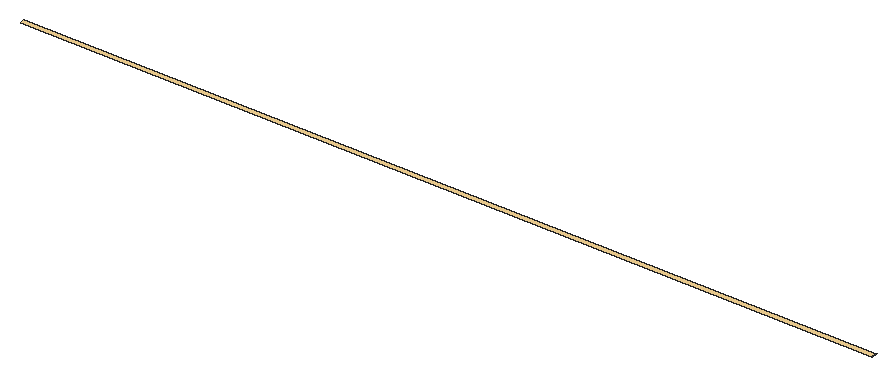
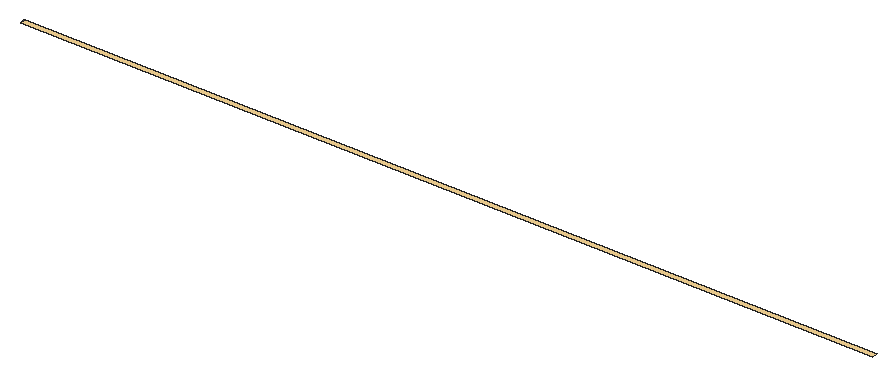
# SketchUp Ruby script. Lengths in inches.
U = 1.inch
M = Sketchup.active_model
def pt(a) = Geom::Point3d.new(a.map { |v| v * U })
def face(e, loops, mat)
  f = e.add_face(loops[0].map { |a| pt(a) })
  loops[1..].each { |l| e.add_face(l.map { |a| pt(a) }).erase! }
  f.material = f.back_material = mat if mat
  f
end
# faces: each face lists its corners as indices into pts; further lists are holes
def faces(e, pts, list, mat = nil) = list.each { |f| face(e, (f[0].is_a?(Array) ? f : [f]).map { |l| l.map { |i| pts[i] } }, mat) }
# xy, xz, yz: faces in a plane at the given z, y or x. An outline is a flat list of corners, or four numbers for a rectangle; further outlines are holes
def ring(l) = l.size == 4 ? [[l[0], l[1]], [l[2], l[1]], [l[2], l[3]], [l[0], l[3]]] : l.each_slice(2).to_a
def flat(e, list, mat, &to3) = list.each { |f| face(e, (f[0].is_a?(Array) ? f : [f]).map { |l| ring(l).map { |u, v| to3.(u, v) } }, mat) }
def xy(e, z, list, mat = nil) = flat(e, list, mat) { |x, y| [x, y, z] }
def xz(e, y, list, mat = nil) = flat(e, list, mat) { |x, z| [x, y, z] }
def yz(e, x, list, mat = nil) = flat(e, list, mat) { |y, z| [x, y, z] }
def lines(e, pts, list) = list.each { |a, b| e.add_line(pt(pts[a]), pt(pts[b])) }
# prism: a flat outline (further loops are holes) pulled along v
def prism(e, loops, v, mat = nil)
  f = face(e, loops, mat); d = Geom::Vector3d.new(v.map { |x| x * U })
  f.pushpull(f.normal.samedirection?(d) ? d.length : -d.length)
end
def box(e, o, s, mat = nil) = prism(e, [[o, [o[0] + s[0], o[1], o[2]], [o[0] + s[0], o[1] + s[1], o[2]], [o[0], o[1] + s[1], o[2]]]], [0, 0, s[2]], mat)
def at(x, y, z, deg = 0) = Geom::Transformation.translation(pt([x, y, z])) * Geom::Transformation.rotation(ORIGIN, Z_AXIS, deg.degrees)
def axes(o, x, y, z) = Geom::Transformation.new([*x, 0, *y, 0, *z, 0, *pt(o).to_a, 1])
def part(name) = M.definitions.add(name)
# library, detail: a bought-in or finely detailed component or shape, given as its bounding box
def library(name, o, s) = part(name).tap { |d| box(d.entities, o, s) }
def detail(e, o, s) = box(e.add_group.entities, o, s)
def put(e, d, t, mat = nil) = e.add_instance(d, t).tap { |i| i.material = mat if mat }
def group(e, t, mat = nil) = e.add_group.tap { |g| g.transformation = t; g.material = mat if mat }.entities
root = M.entities
M.materials.add("1432 AP 8245 TAR ROAD").color = [71, 72, 75]
M.materials.add("Outer Light").color = [251, 217, 152]
xy(root,171.29,[[537,95.37,537.16,96.87]],"1432 AP 8245 TAR ROAD")
xy(root,171.29,[[279,95.37,537,96.87],[537,95.37,537.16,96.87]],"Outer Light")
